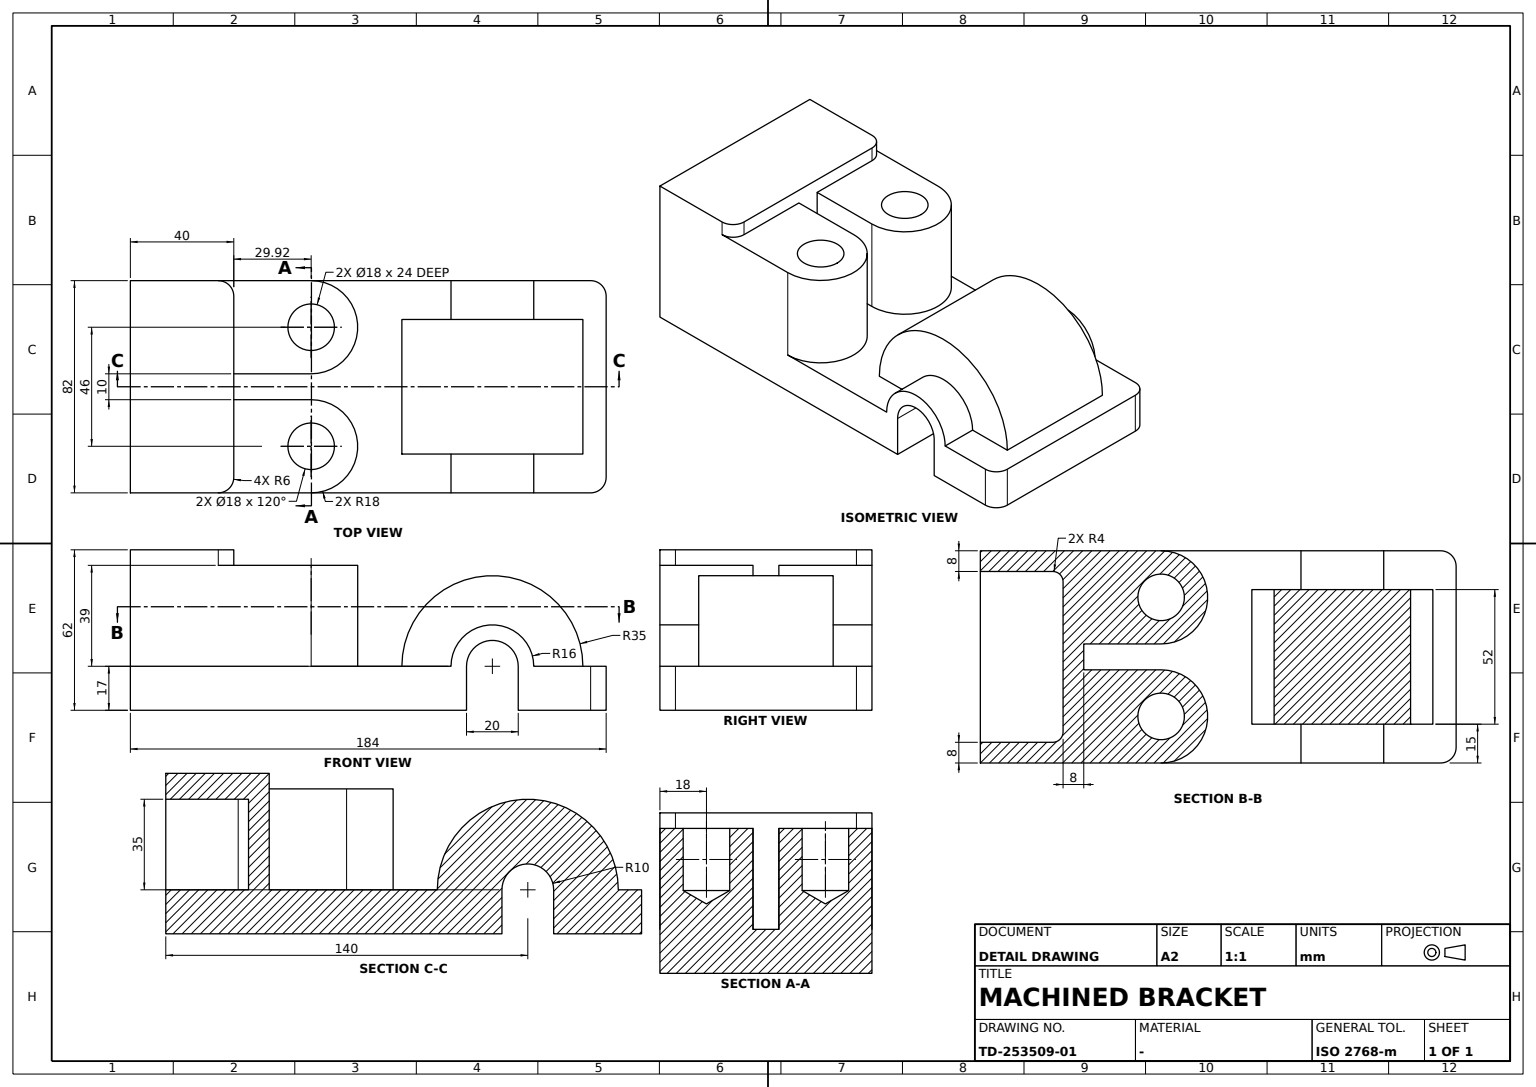
ISO-10303-21;
HEADER;
FILE_DESCRIPTION((''),'2;1');
FILE_NAME('','',(''),(''),'','','');
FILE_SCHEMA(('AUTOMOTIVE_DESIGN'));
ENDSEC;
DATA;
#1=APPLICATION_CONTEXT('');
#2=PRODUCT_CONTEXT('',#1,'mechanical');
#3=PRODUCT('','','',(#2));
#4=PRODUCT_DEFINITION_FORMATION('','',#3);
#5=PRODUCT_DEFINITION_CONTEXT('',#1,'design');
#6=PRODUCT_DEFINITION('','',#4,#5);
#7=PRODUCT_DEFINITION_SHAPE('','',#6);
#8=(LENGTH_UNIT()NAMED_UNIT(*)SI_UNIT(.MILLI.,.METRE.));
#9=(NAMED_UNIT(*)PLANE_ANGLE_UNIT()SI_UNIT($,.RADIAN.));
#10=(NAMED_UNIT(*)SI_UNIT($,.STERADIAN.)SOLID_ANGLE_UNIT());
#11=UNCERTAINTY_MEASURE_WITH_UNIT(LENGTH_MEASURE(0.005),#8,'distance_accuracy_value','');
#12=(GEOMETRIC_REPRESENTATION_CONTEXT(3)GLOBAL_UNCERTAINTY_ASSIGNED_CONTEXT((#11))GLOBAL_UNIT_ASSIGNED_CONTEXT((#8,#9,#10))REPRESENTATION_CONTEXT('',''));
#13=CARTESIAN_POINT('',(10.,-41.,0.));
#14=VERTEX_POINT('',#13);
#15=CARTESIAN_POINT('',(10.,-41.,-17.));
#16=VERTEX_POINT('',#15);
#17=DIRECTION('',(0.,0.,-1.));
#18=VECTOR('',#17,1000.);
#19=LINE('',#13,#18);
#20=EDGE_CURVE('',#14,#16,#19,.T.);
#21=ORIENTED_EDGE('',*,*,#20,.F.);
#22=CARTESIAN_POINT('',(10.,41.,0.));
#23=VERTEX_POINT('',#22);
#24=CARTESIAN_POINT('',(10.,0.,0.));
#25=DIRECTION('',(0.,1.,0.));
#26=VECTOR('',#25,1000.);
#27=LINE('',#24,#26);
#28=EDGE_CURVE('',#14,#23,#27,.T.);
#29=ORIENTED_EDGE('',*,*,#28,.T.);
#30=CARTESIAN_POINT('',(10.,41.,-17.));
#31=VERTEX_POINT('',#30);
#32=LINE('',#22,#18);
#33=EDGE_CURVE('',#23,#31,#32,.T.);
#34=ORIENTED_EDGE('',*,*,#33,.T.);
#35=CARTESIAN_POINT('',(10.,0.,-17.));
#36=LINE('',#35,#26);
#37=EDGE_CURVE('',#16,#31,#36,.T.);
#38=ORIENTED_EDGE('',*,*,#37,.F.);
#39=EDGE_LOOP('',(#21,#29,#34,#38));
#40=FACE_BOUND('',#39,.T.);
#41=DIRECTION('',(1.,0.,0.));
#42=AXIS2_PLACEMENT_3D('',#24,#41,#17);
#43=PLANE('',#42);
#44=ADVANCED_FACE('',(#40),#43,.F.);
#45=CARTESIAN_POINT('',(-16.,26.,0.));
#46=VERTEX_POINT('',#45);
#47=CARTESIAN_POINT('',(-16.,41.,0.));
#48=VERTEX_POINT('',#47);
#49=LINE('',#45,#26);
#50=EDGE_CURVE('',#46,#48,#49,.T.);
#51=ORIENTED_EDGE('',*,*,#50,.F.);
#52=CARTESIAN_POINT('',(16.,26.,0.));
#53=VERTEX_POINT('',#52);
#54=CARTESIAN_POINT('',(0.,26.,0.));
#55=DIRECTION('',(0.,0.,1.));
#56=AXIS2_PLACEMENT_3D('',#54,#25,#55);
#57=CIRCLE('',#56,16.);
#58=EDGE_CURVE('',#46,#53,#57,.T.);
#59=ORIENTED_EDGE('',*,*,#58,.T.);
#60=CARTESIAN_POINT('',(16.,41.,0.));
#61=VERTEX_POINT('',#60);
#62=LINE('',#52,#26);
#63=EDGE_CURVE('',#53,#61,#62,.T.);
#64=ORIENTED_EDGE('',*,*,#63,.T.);
#65=CARTESIAN_POINT('',(0.,41.,0.));
#66=AXIS2_PLACEMENT_3D('',#65,#25,#55);
#67=CIRCLE('',#66,16.);
#68=EDGE_CURVE('',#48,#61,#67,.T.);
#69=ORIENTED_EDGE('',*,*,#68,.F.);
#70=EDGE_LOOP('',(#51,#59,#64,#69));
#71=FACE_BOUND('',#70,.T.);
#72=CARTESIAN_POINT('',(0.,0.,0.));
#73=DIRECTION('',(-1.,0.,0.));
#74=AXIS2_PLACEMENT_3D('',#72,#25,#73);
#75=CYLINDRICAL_SURFACE('',#74,16.);
#76=ADVANCED_FACE('',(#71),#75,.T.);
#77=CARTESIAN_POINT('',(-70.080651,-5.,39.));
#78=VERTEX_POINT('',#77);
#79=CARTESIAN_POINT('',(-100.,-5.,39.));
#80=VERTEX_POINT('',#79);
#81=CARTESIAN_POINT('',(0.,-5.,39.));
#82=VECTOR('',#73,1000.);
#83=LINE('',#81,#82);
#84=EDGE_CURVE('',#78,#80,#83,.T.);
#85=ORIENTED_EDGE('',*,*,#84,.F.);
#86=CARTESIAN_POINT('',(-70.080651,-5.,0.));
#87=VERTEX_POINT('',#86);
#88=CARTESIAN_POINT('',(-70.080651,-5.,19.5));
#89=VECTOR('',#55,1000.);
#90=LINE('',#88,#89);
#91=EDGE_CURVE('',#87,#78,#90,.T.);
#92=ORIENTED_EDGE('',*,*,#91,.F.);
#93=CARTESIAN_POINT('',(-100.,-5.,0.));
#94=VERTEX_POINT('',#93);
#95=LINE('',#86,#82);
#96=EDGE_CURVE('',#87,#94,#95,.T.);
#97=ORIENTED_EDGE('',*,*,#96,.T.);
#98=CARTESIAN_POINT('',(-100.,-5.,45.));
#99=LINE('',#98,#89);
#100=EDGE_CURVE('',#94,#80,#99,.T.);
#101=ORIENTED_EDGE('',*,*,#100,.T.);
#102=EDGE_LOOP('',(#85,#92,#97,#101));
#103=FACE_BOUND('',#102,.T.);
#104=AXIS2_PLACEMENT_3D('',#86,#25,#73);
#105=PLANE('',#104);
#106=ADVANCED_FACE('',(#103),#105,.T.);
#107=CARTESIAN_POINT('',(38.,41.,-17.));
#108=VERTEX_POINT('',#107);
#109=CARTESIAN_POINT('',(0.,41.,-17.));
#110=VECTOR('',#41,1000.);
#111=LINE('',#109,#110);
#112=EDGE_CURVE('',#31,#108,#111,.T.);
#113=ORIENTED_EDGE('',*,*,#112,.F.);
#114=ORIENTED_EDGE('',*,*,#33,.F.);
#115=CARTESIAN_POINT('',(-10.,41.,0.));
#116=VERTEX_POINT('',#115);
#117=CIRCLE('',#66,10.);
#118=EDGE_CURVE('',#116,#23,#117,.T.);
#119=ORIENTED_EDGE('',*,*,#118,.F.);
#120=CARTESIAN_POINT('',(-10.,41.,-17.));
#121=VERTEX_POINT('',#120);
#122=LINE('',#115,#18);
#123=EDGE_CURVE('',#116,#121,#122,.T.);
#124=ORIENTED_EDGE('',*,*,#123,.T.);
#125=CARTESIAN_POINT('',(-140.,41.,-17.));
#126=VERTEX_POINT('',#125);
#127=EDGE_CURVE('',#126,#121,#111,.T.);
#128=ORIENTED_EDGE('',*,*,#127,.F.);
#129=CARTESIAN_POINT('',(-140.,41.,45.));
#130=VERTEX_POINT('',#129);
#131=CARTESIAN_POINT('',(-140.,41.,0.));
#132=LINE('',#131,#89);
#133=EDGE_CURVE('',#126,#130,#132,.T.);
#134=ORIENTED_EDGE('',*,*,#133,.T.);
#135=CARTESIAN_POINT('',(-106.,41.,45.));
#136=VERTEX_POINT('',#135);
#137=CARTESIAN_POINT('',(0.,41.,45.));
#138=LINE('',#137,#110);
#139=EDGE_CURVE('',#130,#136,#138,.T.);
#140=ORIENTED_EDGE('',*,*,#139,.T.);
#141=CARTESIAN_POINT('',(-106.,41.,39.));
#142=VERTEX_POINT('',#141);
#143=CARTESIAN_POINT('',(-106.,41.,40.));
#144=LINE('',#143,#89);
#145=EDGE_CURVE('',#136,#142,#144,.F.);
#146=ORIENTED_EDGE('',*,*,#145,.T.);
#147=CARTESIAN_POINT('',(-70.080651,41.,39.));
#148=VERTEX_POINT('',#147);
#149=CARTESIAN_POINT('',(0.,41.,39.));
#150=LINE('',#149,#82);
#151=EDGE_CURVE('',#148,#142,#150,.T.);
#152=ORIENTED_EDGE('',*,*,#151,.F.);
#153=CARTESIAN_POINT('',(-70.080651,41.,0.));
#154=VERTEX_POINT('',#153);
#155=CARTESIAN_POINT('',(-70.080651,41.,19.5));
#156=LINE('',#155,#89);
#157=EDGE_CURVE('',#154,#148,#156,.T.);
#158=ORIENTED_EDGE('',*,*,#157,.F.);
#159=LINE('',#65,#82);
#160=EDGE_CURVE('',#48,#154,#159,.T.);
#161=ORIENTED_EDGE('',*,*,#160,.F.);
#162=ORIENTED_EDGE('',*,*,#68,.T.);
#163=CARTESIAN_POINT('',(38.,41.,0.));
#164=VERTEX_POINT('',#163);
#165=EDGE_CURVE('',#164,#61,#159,.T.);
#166=ORIENTED_EDGE('',*,*,#165,.F.);
#167=CARTESIAN_POINT('',(38.,41.,14.));
#168=LINE('',#167,#18);
#169=EDGE_CURVE('',#164,#108,#168,.T.);
#170=ORIENTED_EDGE('',*,*,#169,.T.);
#171=EDGE_LOOP('',(#113,#114,#119,#124,#128,#134,#140,#146,#152,#158,#161,#162,#166,#170));
#172=FACE_BOUND('',#171,.T.);
#173=AXIS2_PLACEMENT_3D('',#65,#25,#73);
#174=PLANE('',#173);
#175=ADVANCED_FACE('',(#172),#174,.T.);
#176=CARTESIAN_POINT('',(-140.,-33.,35.));
#177=VERTEX_POINT('',#176);
#178=CARTESIAN_POINT('',(-140.,33.,35.));
#179=VERTEX_POINT('',#178);
#180=CARTESIAN_POINT('',(-140.,0.,35.));
#181=LINE('',#180,#26);
#182=EDGE_CURVE('',#177,#179,#181,.T.);
#183=ORIENTED_EDGE('',*,*,#182,.T.);
#184=CARTESIAN_POINT('',(-112.,33.,35.));
#185=VERTEX_POINT('',#184);
#186=LINE('',#178,#110);
#187=EDGE_CURVE('',#179,#185,#186,.T.);
#188=ORIENTED_EDGE('',*,*,#187,.T.);
#189=CARTESIAN_POINT('',(-108.,29.,35.));
#190=VERTEX_POINT('',#189);
#191=CARTESIAN_POINT('',(-112.,29.,35.));
#192=AXIS2_PLACEMENT_3D('',#191,#55,#41);
#193=CIRCLE('',#192,4.);
#194=EDGE_CURVE('',#190,#185,#193,.T.);
#195=ORIENTED_EDGE('',*,*,#194,.F.);
#196=CARTESIAN_POINT('',(-108.,-29.,35.));
#197=VERTEX_POINT('',#196);
#198=DIRECTION('',(0.,-1.,0.));
#199=VECTOR('',#198,1000.);
#200=LINE('',#189,#199);
#201=EDGE_CURVE('',#190,#197,#200,.T.);
#202=ORIENTED_EDGE('',*,*,#201,.T.);
#203=CARTESIAN_POINT('',(-112.,-33.,35.));
#204=VERTEX_POINT('',#203);
#205=CARTESIAN_POINT('',(-112.,-29.,35.));
#206=AXIS2_PLACEMENT_3D('',#205,#55,#41);
#207=CIRCLE('',#206,4.);
#208=EDGE_CURVE('',#204,#197,#207,.T.);
#209=ORIENTED_EDGE('',*,*,#208,.F.);
#210=CARTESIAN_POINT('',(0.,-33.,35.));
#211=LINE('',#210,#110);
#212=EDGE_CURVE('',#177,#204,#211,.T.);
#213=ORIENTED_EDGE('',*,*,#212,.F.);
#214=EDGE_LOOP('',(#183,#188,#195,#202,#209,#213));
#215=FACE_BOUND('',#214,.T.);
#216=CARTESIAN_POINT('',(0.,0.,35.));
#217=AXIS2_PLACEMENT_3D('',#216,#55,#41);
#218=PLANE('',#217);
#219=ADVANCED_FACE('',(#215),#218,.F.);
#220=CARTESIAN_POINT('',(-140.,-41.,45.));
#221=VERTEX_POINT('',#220);
#222=CARTESIAN_POINT('',(-106.,-41.,45.));
#223=VERTEX_POINT('',#222);
#224=CARTESIAN_POINT('',(0.,-41.,45.));
#225=LINE('',#224,#110);
#226=EDGE_CURVE('',#221,#223,#225,.T.);
#227=ORIENTED_EDGE('',*,*,#226,.F.);
#228=CARTESIAN_POINT('',(-140.,-41.,-17.));
#229=VERTEX_POINT('',#228);
#230=CARTESIAN_POINT('',(-140.,-41.,0.));
#231=LINE('',#230,#89);
#232=EDGE_CURVE('',#229,#221,#231,.T.);
#233=ORIENTED_EDGE('',*,*,#232,.F.);
#234=CARTESIAN_POINT('',(-10.,-41.,-17.));
#235=VERTEX_POINT('',#234);
#236=CARTESIAN_POINT('',(0.,-41.,-17.));
#237=LINE('',#236,#110);
#238=EDGE_CURVE('',#229,#235,#237,.T.);
#239=ORIENTED_EDGE('',*,*,#238,.T.);
#240=CARTESIAN_POINT('',(-10.,-41.,0.));
#241=VERTEX_POINT('',#240);
#242=LINE('',#240,#18);
#243=EDGE_CURVE('',#241,#235,#242,.T.);
#244=ORIENTED_EDGE('',*,*,#243,.F.);
#245=CARTESIAN_POINT('',(0.,-41.,0.));
#246=AXIS2_PLACEMENT_3D('',#245,#25,#55);
#247=CIRCLE('',#246,10.);
#248=EDGE_CURVE('',#241,#14,#247,.T.);
#249=ORIENTED_EDGE('',*,*,#248,.T.);
#250=ORIENTED_EDGE('',*,*,#20,.T.);
#251=CARTESIAN_POINT('',(38.,-41.,-17.));
#252=VERTEX_POINT('',#251);
#253=EDGE_CURVE('',#16,#252,#237,.T.);
#254=ORIENTED_EDGE('',*,*,#253,.T.);
#255=CARTESIAN_POINT('',(38.,-41.,0.));
#256=VERTEX_POINT('',#255);
#257=CARTESIAN_POINT('',(38.,-41.,14.));
#258=LINE('',#257,#18);
#259=EDGE_CURVE('',#256,#252,#258,.T.);
#260=ORIENTED_EDGE('',*,*,#259,.F.);
#261=CARTESIAN_POINT('',(16.,-41.,0.));
#262=VERTEX_POINT('',#261);
#263=LINE('',#245,#82);
#264=EDGE_CURVE('',#256,#262,#263,.T.);
#265=ORIENTED_EDGE('',*,*,#264,.T.);
#266=CARTESIAN_POINT('',(-16.,-41.,0.));
#267=VERTEX_POINT('',#266);
#268=CIRCLE('',#246,16.);
#269=EDGE_CURVE('',#267,#262,#268,.T.);
#270=ORIENTED_EDGE('',*,*,#269,.F.);
#271=CARTESIAN_POINT('',(-70.080651,-41.,0.));
#272=VERTEX_POINT('',#271);
#273=EDGE_CURVE('',#267,#272,#263,.T.);
#274=ORIENTED_EDGE('',*,*,#273,.T.);
#275=CARTESIAN_POINT('',(-70.080651,-41.,39.));
#276=VERTEX_POINT('',#275);
#277=CARTESIAN_POINT('',(-70.080651,-41.,19.5));
#278=LINE('',#277,#89);
#279=EDGE_CURVE('',#272,#276,#278,.T.);
#280=ORIENTED_EDGE('',*,*,#279,.T.);
#281=CARTESIAN_POINT('',(-106.,-41.,39.));
#282=VERTEX_POINT('',#281);
#283=CARTESIAN_POINT('',(0.,-41.,39.));
#284=LINE('',#283,#110);
#285=EDGE_CURVE('',#282,#276,#284,.T.);
#286=ORIENTED_EDGE('',*,*,#285,.F.);
#287=CARTESIAN_POINT('',(-106.,-41.,40.));
#288=LINE('',#287,#89);
#289=EDGE_CURVE('',#223,#282,#288,.F.);
#290=ORIENTED_EDGE('',*,*,#289,.F.);
#291=EDGE_LOOP('',(#227,#233,#239,#244,#249,#250,#254,#260,#265,#270,#274,#280,#286,#290));
#292=FACE_BOUND('',#291,.T.);
#293=AXIS2_PLACEMENT_3D('',#245,#25,#73);
#294=PLANE('',#293);
#295=ADVANCED_FACE('',(#292),#294,.F.);
#296=CARTESIAN_POINT('',(-100.,-35.,45.));
#297=VERTEX_POINT('',#296);
#298=CARTESIAN_POINT('',(-106.,-35.,45.));
#299=AXIS2_PLACEMENT_3D('',#298,#55,#41);
#300=CIRCLE('',#299,6.);
#301=EDGE_CURVE('',#223,#297,#300,.T.);
#302=ORIENTED_EDGE('',*,*,#301,.F.);
#303=ORIENTED_EDGE('',*,*,#289,.T.);
#304=CARTESIAN_POINT('',(-100.,-35.,39.));
#305=VERTEX_POINT('',#304);
#306=CARTESIAN_POINT('',(-106.,-35.,39.));
#307=AXIS2_PLACEMENT_3D('',#306,#55,#41);
#308=CIRCLE('',#307,6.);
#309=EDGE_CURVE('',#282,#305,#308,.T.);
#310=ORIENTED_EDGE('',*,*,#309,.T.);
#311=CARTESIAN_POINT('',(-100.,-35.,40.));
#312=LINE('',#311,#89);
#313=EDGE_CURVE('',#297,#305,#312,.F.);
#314=ORIENTED_EDGE('',*,*,#313,.F.);
#315=EDGE_LOOP('',(#302,#303,#310,#314));
#316=FACE_BOUND('',#315,.T.);
#317=CARTESIAN_POINT('',(-106.,-35.,40.));
#318=AXIS2_PLACEMENT_3D('',#317,#55,#41);
#319=CYLINDRICAL_SURFACE('',#318,6.);
#320=ADVANCED_FACE('',(#316),#319,.T.);
#321=CARTESIAN_POINT('',(44.,-35.,0.));
#322=VERTEX_POINT('',#321);
#323=CARTESIAN_POINT('',(44.,35.,0.));
#324=VERTEX_POINT('',#323);
#325=CARTESIAN_POINT('',(44.,0.,0.));
#326=LINE('',#325,#26);
#327=EDGE_CURVE('',#322,#324,#326,.T.);
#328=ORIENTED_EDGE('',*,*,#327,.T.);
#329=CARTESIAN_POINT('',(38.,35.,0.));
#330=AXIS2_PLACEMENT_3D('',#329,#17,#73);
#331=CIRCLE('',#330,6.);
#332=EDGE_CURVE('',#164,#324,#331,.T.);
#333=ORIENTED_EDGE('',*,*,#332,.F.);
#334=ORIENTED_EDGE('',*,*,#165,.T.);
#335=ORIENTED_EDGE('',*,*,#63,.F.);
#336=CARTESIAN_POINT('',(35.,26.,0.));
#337=VERTEX_POINT('',#336);
#338=CARTESIAN_POINT('',(44.,26.,0.));
#339=LINE('',#338,#110);
#340=EDGE_CURVE('',#53,#337,#339,.T.);
#341=ORIENTED_EDGE('',*,*,#340,.T.);
#342=CARTESIAN_POINT('',(35.,-26.,0.));
#343=VERTEX_POINT('',#342);
#344=LINE('',#342,#26);
#345=EDGE_CURVE('',#343,#337,#344,.T.);
#346=ORIENTED_EDGE('',*,*,#345,.F.);
#347=CARTESIAN_POINT('',(16.,-26.,0.));
#348=VERTEX_POINT('',#347);
#349=CARTESIAN_POINT('',(44.,-26.,0.));
#350=LINE('',#349,#110);
#351=EDGE_CURVE('',#348,#343,#350,.T.);
#352=ORIENTED_EDGE('',*,*,#351,.F.);
#353=LINE('',#261,#26);
#354=EDGE_CURVE('',#262,#348,#353,.T.);
#355=ORIENTED_EDGE('',*,*,#354,.F.);
#356=ORIENTED_EDGE('',*,*,#264,.F.);
#357=CARTESIAN_POINT('',(38.,-35.,0.));
#358=AXIS2_PLACEMENT_3D('',#357,#17,#73);
#359=CIRCLE('',#358,6.);
#360=EDGE_CURVE('',#322,#256,#359,.T.);
#361=ORIENTED_EDGE('',*,*,#360,.F.);
#362=EDGE_LOOP('',(#328,#333,#334,#335,#341,#346,#352,#355,#356,#361));
#363=FACE_BOUND('',#362,.T.);
#364=AXIS2_PLACEMENT_3D('',#325,#17,#73);
#365=PLANE('',#364);
#366=ADVANCED_FACE('',(#363),#365,.F.);
#367=ORIENTED_EDGE('',*,*,#58,.F.);
#368=CARTESIAN_POINT('',(-35.,26.,0.));
#369=VERTEX_POINT('',#368);
#370=LINE('',#54,#82);
#371=EDGE_CURVE('',#46,#369,#370,.T.);
#372=ORIENTED_EDGE('',*,*,#371,.T.);
#373=CIRCLE('',#56,35.);
#374=EDGE_CURVE('',#369,#337,#373,.T.);
#375=ORIENTED_EDGE('',*,*,#374,.T.);
#376=ORIENTED_EDGE('',*,*,#340,.F.);
#377=EDGE_LOOP('',(#367,#372,#375,#376));
#378=FACE_BOUND('',#377,.T.);
#379=AXIS2_PLACEMENT_3D('',#54,#25,#73);
#380=PLANE('',#379);
#381=ADVANCED_FACE('',(#378),#380,.T.);
#382=ORIENTED_EDGE('',*,*,#212,.T.);
#383=CARTESIAN_POINT('',(-112.,-33.,0.));
#384=VERTEX_POINT('',#383);
#385=CARTESIAN_POINT('',(-112.,-33.,22.5));
#386=LINE('',#385,#89);
#387=EDGE_CURVE('',#204,#384,#386,.F.);
#388=ORIENTED_EDGE('',*,*,#387,.T.);
#389=CARTESIAN_POINT('',(-140.,-33.,0.));
#390=VERTEX_POINT('',#389);
#391=CARTESIAN_POINT('',(44.,-33.,0.));
#392=LINE('',#391,#82);
#393=EDGE_CURVE('',#384,#390,#392,.T.);
#394=ORIENTED_EDGE('',*,*,#393,.T.);
#395=CARTESIAN_POINT('',(-140.,-33.,45.));
#396=LINE('',#395,#18);
#397=EDGE_CURVE('',#177,#390,#396,.T.);
#398=ORIENTED_EDGE('',*,*,#397,.F.);
#399=EDGE_LOOP('',(#382,#388,#394,#398));
#400=FACE_BOUND('',#399,.T.);
#401=CARTESIAN_POINT('',(-112.,-33.,45.));
#402=AXIS2_PLACEMENT_3D('',#401,#198,#73);
#403=PLANE('',#402);
#404=ADVANCED_FACE('',(#400),#403,.F.);
#405=CARTESIAN_POINT('',(-108.,29.,0.));
#406=VERTEX_POINT('',#405);
#407=CARTESIAN_POINT('',(-108.,29.,22.5));
#408=LINE('',#407,#89);
#409=EDGE_CURVE('',#190,#406,#408,.F.);
#410=ORIENTED_EDGE('',*,*,#409,.F.);
#411=ORIENTED_EDGE('',*,*,#194,.T.);
#412=CARTESIAN_POINT('',(-112.,33.,0.));
#413=VERTEX_POINT('',#412);
#414=CARTESIAN_POINT('',(-112.,33.,22.5));
#415=LINE('',#414,#89);
#416=EDGE_CURVE('',#185,#413,#415,.F.);
#417=ORIENTED_EDGE('',*,*,#416,.T.);
#418=CARTESIAN_POINT('',(-112.,29.,0.));
#419=AXIS2_PLACEMENT_3D('',#418,#17,#73);
#420=CIRCLE('',#419,4.);
#421=EDGE_CURVE('',#406,#413,#420,.F.);
#422=ORIENTED_EDGE('',*,*,#421,.F.);
#423=EDGE_LOOP('',(#410,#411,#417,#422));
#424=FACE_BOUND('',#423,.T.);
#425=CARTESIAN_POINT('',(-112.,29.,22.5));
#426=AXIS2_PLACEMENT_3D('',#425,#55,#41);
#427=CYLINDRICAL_SURFACE('',#426,4.);
#428=ADVANCED_FACE('',(#424),#427,.F.);
#429=ORIENTED_EDGE('',*,*,#397,.T.);
#430=CARTESIAN_POINT('',(-140.,33.,0.));
#431=VERTEX_POINT('',#430);
#432=CARTESIAN_POINT('',(-140.,0.,0.));
#433=LINE('',#432,#199);
#434=EDGE_CURVE('',#431,#390,#433,.T.);
#435=ORIENTED_EDGE('',*,*,#434,.F.);
#436=CARTESIAN_POINT('',(-140.,33.,-17.));
#437=LINE('',#436,#18);
#438=EDGE_CURVE('',#179,#431,#437,.T.);
#439=ORIENTED_EDGE('',*,*,#438,.F.);
#440=ORIENTED_EDGE('',*,*,#182,.F.);
#441=EDGE_LOOP('',(#429,#435,#439,#440));
#442=FACE_BOUND('',#441,.T.);
#443=CARTESIAN_POINT('',(-140.,0.,-17.));
#444=LINE('',#443,#26);
#445=EDGE_CURVE('',#229,#126,#444,.T.);
#446=ORIENTED_EDGE('',*,*,#445,.F.);
#447=ORIENTED_EDGE('',*,*,#232,.T.);
#448=CARTESIAN_POINT('',(-140.,0.,45.));
#449=LINE('',#448,#26);
#450=EDGE_CURVE('',#221,#130,#449,.T.);
#451=ORIENTED_EDGE('',*,*,#450,.T.);
#452=ORIENTED_EDGE('',*,*,#133,.F.);
#453=EDGE_LOOP('',(#446,#447,#451,#452));
#454=FACE_BOUND('',#453,.T.);
#455=AXIS2_PLACEMENT_3D('',#443,#73,#55);
#456=PLANE('',#455);
#457=ADVANCED_FACE('',(#442,#454),#456,.T.);
#458=CARTESIAN_POINT('',(-100.,35.,45.));
#459=VERTEX_POINT('',#458);
#460=CARTESIAN_POINT('',(-100.,35.,39.));
#461=VERTEX_POINT('',#460);
#462=CARTESIAN_POINT('',(-100.,35.,40.));
#463=LINE('',#462,#89);
#464=EDGE_CURVE('',#459,#461,#463,.F.);
#465=ORIENTED_EDGE('',*,*,#464,.T.);
#466=CARTESIAN_POINT('',(-106.,35.,39.));
#467=AXIS2_PLACEMENT_3D('',#466,#55,#41);
#468=CIRCLE('',#467,6.);
#469=EDGE_CURVE('',#461,#142,#468,.T.);
#470=ORIENTED_EDGE('',*,*,#469,.T.);
#471=ORIENTED_EDGE('',*,*,#145,.F.);
#472=CARTESIAN_POINT('',(-106.,35.,45.));
#473=AXIS2_PLACEMENT_3D('',#472,#55,#41);
#474=CIRCLE('',#473,6.);
#475=EDGE_CURVE('',#459,#136,#474,.T.);
#476=ORIENTED_EDGE('',*,*,#475,.F.);
#477=EDGE_LOOP('',(#465,#470,#471,#476));
#478=FACE_BOUND('',#477,.T.);
#479=CARTESIAN_POINT('',(-106.,35.,40.));
#480=AXIS2_PLACEMENT_3D('',#479,#55,#41);
#481=CYLINDRICAL_SURFACE('',#480,6.);
#482=ADVANCED_FACE('',(#478),#481,.T.);
#483=CARTESIAN_POINT('',(-61.080651,-23.,15.));
#484=VERTEX_POINT('',#483);
#485=CARTESIAN_POINT('',(-70.080651,-23.,15.));
#486=AXIS2_PLACEMENT_3D('',#485,#55,#41);
#487=CIRCLE('',#486,9.);
#488=EDGE_CURVE('',#484,#484,#487,.F.);
#489=ORIENTED_EDGE('',*,*,#488,.F.);
#490=EDGE_LOOP('',(#489));
#491=FACE_BOUND('',#490,.T.);
#492=CARTESIAN_POINT('',(-70.080651,-23.,9.803848));
#493=VERTEX_POINT('',#492);
#494=VERTEX_LOOP('',#493);
#495=FACE_BOUND('',#494,.T.);
#496=AXIS2_PLACEMENT_3D('',#492,#55,#41);
#497=CONICAL_SURFACE('',#496,0.,1.047197551);
#498=ADVANCED_FACE('',(#491,#495),#497,.F.);
#499=ORIENTED_EDGE('',*,*,#243,.T.);
#500=CARTESIAN_POINT('',(-10.,0.,-17.));
#501=LINE('',#500,#26);
#502=EDGE_CURVE('',#235,#121,#501,.T.);
#503=ORIENTED_EDGE('',*,*,#502,.T.);
#504=ORIENTED_EDGE('',*,*,#123,.F.);
#505=CARTESIAN_POINT('',(-10.,0.,0.));
#506=LINE('',#505,#26);
#507=EDGE_CURVE('',#241,#116,#506,.T.);
#508=ORIENTED_EDGE('',*,*,#507,.F.);
#509=EDGE_LOOP('',(#499,#503,#504,#508));
#510=FACE_BOUND('',#509,.T.);
#511=AXIS2_PLACEMENT_3D('',#505,#41,#17);
#512=PLANE('',#511);
#513=ADVANCED_FACE('',(#510),#512,.T.);
#514=ORIENTED_EDGE('',*,*,#332,.T.);
#515=CARTESIAN_POINT('',(44.,35.,-17.));
#516=VERTEX_POINT('',#515);
#517=CARTESIAN_POINT('',(44.,35.,14.));
#518=LINE('',#517,#18);
#519=EDGE_CURVE('',#324,#516,#518,.T.);
#520=ORIENTED_EDGE('',*,*,#519,.T.);
#521=CARTESIAN_POINT('',(38.,35.,-17.));
#522=AXIS2_PLACEMENT_3D('',#521,#55,#41);
#523=CIRCLE('',#522,6.);
#524=EDGE_CURVE('',#516,#108,#523,.T.);
#525=ORIENTED_EDGE('',*,*,#524,.T.);
#526=ORIENTED_EDGE('',*,*,#169,.F.);
#527=EDGE_LOOP('',(#514,#520,#525,#526));
#528=FACE_BOUND('',#527,.T.);
#529=CARTESIAN_POINT('',(38.,35.,14.));
#530=AXIS2_PLACEMENT_3D('',#529,#17,#41);
#531=CYLINDRICAL_SURFACE('',#530,6.);
#532=ADVANCED_FACE('',(#528),#531,.T.);
#533=CARTESIAN_POINT('',(-70.080651,5.,0.));
#534=VERTEX_POINT('',#533);
#535=CARTESIAN_POINT('',(-70.080651,23.,0.));
#536=AXIS2_PLACEMENT_3D('',#535,#17,#73);
#537=CIRCLE('',#536,18.);
#538=EDGE_CURVE('',#534,#154,#537,.F.);
#539=ORIENTED_EDGE('',*,*,#538,.T.);
#540=ORIENTED_EDGE('',*,*,#157,.T.);
#541=CARTESIAN_POINT('',(-70.080651,5.,39.));
#542=VERTEX_POINT('',#541);
#543=CARTESIAN_POINT('',(-70.080651,23.,39.));
#544=AXIS2_PLACEMENT_3D('',#543,#55,#41);
#545=CIRCLE('',#544,18.);
#546=EDGE_CURVE('',#542,#148,#545,.T.);
#547=ORIENTED_EDGE('',*,*,#546,.F.);
#548=CARTESIAN_POINT('',(-70.080651,5.,19.5));
#549=LINE('',#548,#89);
#550=EDGE_CURVE('',#534,#542,#549,.T.);
#551=ORIENTED_EDGE('',*,*,#550,.F.);
#552=EDGE_LOOP('',(#539,#540,#547,#551));
#553=FACE_BOUND('',#552,.T.);
#554=CARTESIAN_POINT('',(-70.080651,23.,19.5));
#555=AXIS2_PLACEMENT_3D('',#554,#55,#41);
#556=CYLINDRICAL_SURFACE('',#555,18.);
#557=ADVANCED_FACE('',(#553),#556,.T.);
#558=CARTESIAN_POINT('',(-61.080651,23.,15.));
#559=VERTEX_POINT('',#558);
#560=CARTESIAN_POINT('',(-70.080651,23.,15.));
#561=AXIS2_PLACEMENT_3D('',#560,#55,#41);
#562=CIRCLE('',#561,9.);
#563=EDGE_CURVE('',#559,#559,#562,.F.);
#564=ORIENTED_EDGE('',*,*,#563,.T.);
#565=EDGE_LOOP('',(#564));
#566=FACE_BOUND('',#565,.T.);
#567=CARTESIAN_POINT('',(-61.080651,23.,39.));
#568=VERTEX_POINT('',#567);
#569=CIRCLE('',#544,9.);
#570=EDGE_CURVE('',#568,#568,#569,.T.);
#571=ORIENTED_EDGE('',*,*,#570,.T.);
#572=EDGE_LOOP('',(#571));
#573=FACE_BOUND('',#572,.T.);
#574=CARTESIAN_POINT('',(-70.080651,23.,38.9));
#575=AXIS2_PLACEMENT_3D('',#574,#17,#41);
#576=CYLINDRICAL_SURFACE('',#575,9.);
#577=ADVANCED_FACE('',(#566,#573),#576,.F.);
#578=ORIENTED_EDGE('',*,*,#570,.F.);
#579=EDGE_LOOP('',(#578));
#580=FACE_BOUND('',#579,.T.);
#581=ORIENTED_EDGE('',*,*,#469,.F.);
#582=CARTESIAN_POINT('',(-100.,5.,39.));
#583=VERTEX_POINT('',#582);
#584=CARTESIAN_POINT('',(-100.,0.,39.));
#585=LINE('',#584,#26);
#586=EDGE_CURVE('',#583,#461,#585,.T.);
#587=ORIENTED_EDGE('',*,*,#586,.F.);
#588=CARTESIAN_POINT('',(0.,5.,39.));
#589=LINE('',#588,#82);
#590=EDGE_CURVE('',#542,#583,#589,.T.);
#591=ORIENTED_EDGE('',*,*,#590,.F.);
#592=ORIENTED_EDGE('',*,*,#546,.T.);
#593=ORIENTED_EDGE('',*,*,#151,.T.);
#594=EDGE_LOOP('',(#581,#587,#591,#592,#593));
#595=FACE_BOUND('',#594,.T.);
#596=CARTESIAN_POINT('',(0.,0.,39.));
#597=AXIS2_PLACEMENT_3D('',#596,#55,#41);
#598=PLANE('',#597);
#599=ADVANCED_FACE('',(#580,#595),#598,.T.);
#600=ORIENTED_EDGE('',*,*,#507,.T.);
#601=ORIENTED_EDGE('',*,*,#118,.T.);
#602=ORIENTED_EDGE('',*,*,#28,.F.);
#603=ORIENTED_EDGE('',*,*,#248,.F.);
#604=EDGE_LOOP('',(#600,#601,#602,#603));
#605=FACE_BOUND('',#604,.T.);
#606=CYLINDRICAL_SURFACE('',#74,10.);
#607=ADVANCED_FACE('',(#605),#606,.F.);
#608=CARTESIAN_POINT('',(-61.080651,-23.,39.));
#609=VERTEX_POINT('',#608);
#610=CARTESIAN_POINT('',(-70.080651,-23.,39.));
#611=AXIS2_PLACEMENT_3D('',#610,#55,#41);
#612=CIRCLE('',#611,9.);
#613=EDGE_CURVE('',#609,#609,#612,.T.);
#614=ORIENTED_EDGE('',*,*,#613,.T.);
#615=EDGE_LOOP('',(#614));
#616=FACE_BOUND('',#615,.T.);
#617=ORIENTED_EDGE('',*,*,#488,.T.);
#618=EDGE_LOOP('',(#617));
#619=FACE_BOUND('',#618,.T.);
#620=CARTESIAN_POINT('',(-70.080651,-23.,38.9));
#621=AXIS2_PLACEMENT_3D('',#620,#17,#41);
#622=CYLINDRICAL_SURFACE('',#621,9.);
#623=ADVANCED_FACE('',(#616,#619),#622,.F.);
#624=ORIENTED_EDGE('',*,*,#226,.T.);
#625=ORIENTED_EDGE('',*,*,#301,.T.);
#626=CARTESIAN_POINT('',(-100.,0.,45.));
#627=LINE('',#626,#26);
#628=EDGE_CURVE('',#297,#459,#627,.T.);
#629=ORIENTED_EDGE('',*,*,#628,.T.);
#630=ORIENTED_EDGE('',*,*,#475,.T.);
#631=ORIENTED_EDGE('',*,*,#139,.F.);
#632=ORIENTED_EDGE('',*,*,#450,.F.);
#633=EDGE_LOOP('',(#624,#625,#629,#630,#631,#632));
#634=FACE_BOUND('',#633,.T.);
#635=AXIS2_PLACEMENT_3D('',#448,#55,#41);
#636=PLANE('',#635);
#637=ADVANCED_FACE('',(#634),#636,.T.);
#638=ORIENTED_EDGE('',*,*,#37,.T.);
#639=ORIENTED_EDGE('',*,*,#112,.T.);
#640=ORIENTED_EDGE('',*,*,#524,.F.);
#641=CARTESIAN_POINT('',(44.,-35.,-17.));
#642=VERTEX_POINT('',#641);
#643=CARTESIAN_POINT('',(44.,0.,-17.));
#644=LINE('',#643,#26);
#645=EDGE_CURVE('',#642,#516,#644,.T.);
#646=ORIENTED_EDGE('',*,*,#645,.F.);
#647=CARTESIAN_POINT('',(38.,-35.,-17.));
#648=AXIS2_PLACEMENT_3D('',#647,#55,#41);
#649=CIRCLE('',#648,6.);
#650=EDGE_CURVE('',#252,#642,#649,.T.);
#651=ORIENTED_EDGE('',*,*,#650,.F.);
#652=ORIENTED_EDGE('',*,*,#253,.F.);
#653=EDGE_LOOP('',(#638,#639,#640,#646,#651,#652));
#654=FACE_BOUND('',#653,.T.);
#655=AXIS2_PLACEMENT_3D('',#35,#55,#41);
#656=PLANE('',#655);
#657=ADVANCED_FACE('',(#654),#656,.F.);
#658=EDGE_CURVE('',#305,#80,#585,.T.);
#659=ORIENTED_EDGE('',*,*,#658,.T.);
#660=ORIENTED_EDGE('',*,*,#100,.F.);
#661=CARTESIAN_POINT('',(-100.,5.,0.));
#662=VERTEX_POINT('',#661);
#663=CARTESIAN_POINT('',(-100.,0.,0.));
#664=LINE('',#663,#26);
#665=EDGE_CURVE('',#94,#662,#664,.T.);
#666=ORIENTED_EDGE('',*,*,#665,.T.);
#667=CARTESIAN_POINT('',(-100.,5.,45.));
#668=LINE('',#667,#89);
#669=EDGE_CURVE('',#662,#583,#668,.T.);
#670=ORIENTED_EDGE('',*,*,#669,.T.);
#671=ORIENTED_EDGE('',*,*,#586,.T.);
#672=ORIENTED_EDGE('',*,*,#464,.F.);
#673=ORIENTED_EDGE('',*,*,#628,.F.);
#674=ORIENTED_EDGE('',*,*,#313,.T.);
#675=EDGE_LOOP('',(#659,#660,#666,#670,#671,#672,#673,#674));
#676=FACE_BOUND('',#675,.T.);
#677=AXIS2_PLACEMENT_3D('',#626,#41,#17);
#678=PLANE('',#677);
#679=ADVANCED_FACE('',(#676),#678,.T.);
#680=ORIENTED_EDGE('',*,*,#285,.T.);
#681=CIRCLE('',#611,18.);
#682=EDGE_CURVE('',#276,#78,#681,.T.);
#683=ORIENTED_EDGE('',*,*,#682,.T.);
#684=ORIENTED_EDGE('',*,*,#84,.T.);
#685=ORIENTED_EDGE('',*,*,#658,.F.);
#686=ORIENTED_EDGE('',*,*,#309,.F.);
#687=EDGE_LOOP('',(#680,#683,#684,#685,#686));
#688=FACE_BOUND('',#687,.T.);
#689=ORIENTED_EDGE('',*,*,#613,.F.);
#690=EDGE_LOOP('',(#689));
#691=FACE_BOUND('',#690,.T.);
#692=ADVANCED_FACE('',(#688,#691),#598,.T.);
#693=ORIENTED_EDGE('',*,*,#354,.T.);
#694=CARTESIAN_POINT('',(-16.,-26.,0.));
#695=VERTEX_POINT('',#694);
#696=CARTESIAN_POINT('',(0.,-26.,0.));
#697=AXIS2_PLACEMENT_3D('',#696,#25,#55);
#698=CIRCLE('',#697,16.);
#699=EDGE_CURVE('',#695,#348,#698,.T.);
#700=ORIENTED_EDGE('',*,*,#699,.F.);
#701=LINE('',#266,#26);
#702=EDGE_CURVE('',#267,#695,#701,.T.);
#703=ORIENTED_EDGE('',*,*,#702,.F.);
#704=ORIENTED_EDGE('',*,*,#269,.T.);
#705=EDGE_LOOP('',(#693,#700,#703,#704));
#706=FACE_BOUND('',#705,.T.);
#707=ADVANCED_FACE('',(#706),#75,.T.);
#708=ORIENTED_EDGE('',*,*,#327,.F.);
#709=CARTESIAN_POINT('',(44.,-35.,14.));
#710=LINE('',#709,#18);
#711=EDGE_CURVE('',#322,#642,#710,.T.);
#712=ORIENTED_EDGE('',*,*,#711,.T.);
#713=ORIENTED_EDGE('',*,*,#645,.T.);
#714=ORIENTED_EDGE('',*,*,#519,.F.);
#715=EDGE_LOOP('',(#708,#712,#713,#714));
#716=FACE_BOUND('',#715,.T.);
#717=AXIS2_PLACEMENT_3D('',#325,#41,#17);
#718=PLANE('',#717);
#719=ADVANCED_FACE('',(#716),#718,.T.);
#720=CARTESIAN_POINT('',(-108.,-29.,0.));
#721=VERTEX_POINT('',#720);
#722=CARTESIAN_POINT('',(-108.,0.,0.));
#723=LINE('',#722,#199);
#724=EDGE_CURVE('',#406,#721,#723,.T.);
#725=ORIENTED_EDGE('',*,*,#724,.F.);
#726=ORIENTED_EDGE('',*,*,#421,.T.);
#727=CARTESIAN_POINT('',(44.,33.,0.));
#728=LINE('',#727,#110);
#729=EDGE_CURVE('',#431,#413,#728,.T.);
#730=ORIENTED_EDGE('',*,*,#729,.F.);
#731=ORIENTED_EDGE('',*,*,#434,.T.);
#732=ORIENTED_EDGE('',*,*,#393,.F.);
#733=CARTESIAN_POINT('',(-112.,-29.,0.));
#734=AXIS2_PLACEMENT_3D('',#733,#17,#73);
#735=CIRCLE('',#734,4.);
#736=EDGE_CURVE('',#384,#721,#735,.F.);
#737=ORIENTED_EDGE('',*,*,#736,.T.);
#738=EDGE_LOOP('',(#725,#726,#730,#731,#732,#737));
#739=FACE_BOUND('',#738,.T.);
#740=ADVANCED_FACE('',(#739),#365,.F.);
#741=ORIENTED_EDGE('',*,*,#371,.F.);
#742=ORIENTED_EDGE('',*,*,#50,.T.);
#743=ORIENTED_EDGE('',*,*,#160,.T.);
#744=ORIENTED_EDGE('',*,*,#538,.F.);
#745=LINE('',#533,#82);
#746=EDGE_CURVE('',#534,#662,#745,.T.);
#747=ORIENTED_EDGE('',*,*,#746,.T.);
#748=ORIENTED_EDGE('',*,*,#665,.F.);
#749=ORIENTED_EDGE('',*,*,#96,.F.);
#750=CARTESIAN_POINT('',(-70.080651,-23.,0.));
#751=AXIS2_PLACEMENT_3D('',#750,#17,#73);
#752=CIRCLE('',#751,18.);
#753=EDGE_CURVE('',#272,#87,#752,.F.);
#754=ORIENTED_EDGE('',*,*,#753,.F.);
#755=ORIENTED_EDGE('',*,*,#273,.F.);
#756=ORIENTED_EDGE('',*,*,#702,.T.);
#757=CARTESIAN_POINT('',(-35.,-26.,0.));
#758=VERTEX_POINT('',#757);
#759=LINE('',#696,#82);
#760=EDGE_CURVE('',#695,#758,#759,.T.);
#761=ORIENTED_EDGE('',*,*,#760,.T.);
#762=LINE('',#757,#26);
#763=EDGE_CURVE('',#758,#369,#762,.T.);
#764=ORIENTED_EDGE('',*,*,#763,.T.);
#765=EDGE_LOOP('',(#741,#742,#743,#744,#747,#748,#749,#754,#755,#756,#761,#764));
#766=FACE_BOUND('',#765,.T.);
#767=ADVANCED_FACE('',(#766),#365,.F.);
#768=ORIENTED_EDGE('',*,*,#279,.F.);
#769=ORIENTED_EDGE('',*,*,#753,.T.);
#770=ORIENTED_EDGE('',*,*,#91,.T.);
#771=ORIENTED_EDGE('',*,*,#682,.F.);
#772=EDGE_LOOP('',(#768,#769,#770,#771));
#773=FACE_BOUND('',#772,.T.);
#774=CARTESIAN_POINT('',(-70.080651,-23.,19.5));
#775=AXIS2_PLACEMENT_3D('',#774,#55,#41);
#776=CYLINDRICAL_SURFACE('',#775,18.);
#777=ADVANCED_FACE('',(#773),#776,.T.);
#778=ORIENTED_EDGE('',*,*,#724,.T.);
#779=CARTESIAN_POINT('',(-108.,-29.,22.5));
#780=LINE('',#779,#89);
#781=EDGE_CURVE('',#197,#721,#780,.F.);
#782=ORIENTED_EDGE('',*,*,#781,.F.);
#783=ORIENTED_EDGE('',*,*,#201,.F.);
#784=ORIENTED_EDGE('',*,*,#409,.T.);
#785=EDGE_LOOP('',(#778,#782,#783,#784));
#786=FACE_BOUND('',#785,.T.);
#787=CARTESIAN_POINT('',(-108.,29.,45.));
#788=AXIS2_PLACEMENT_3D('',#787,#41,#198);
#789=PLANE('',#788);
#790=ADVANCED_FACE('',(#786),#789,.F.);
#791=CARTESIAN_POINT('',(-70.080651,23.,9.803848));
#792=VERTEX_POINT('',#791);
#793=VERTEX_LOOP('',#792);
#794=FACE_BOUND('',#793,.T.);
#795=ORIENTED_EDGE('',*,*,#563,.F.);
#796=EDGE_LOOP('',(#795));
#797=FACE_BOUND('',#796,.T.);
#798=AXIS2_PLACEMENT_3D('',#791,#55,#41);
#799=CONICAL_SURFACE('',#798,0.,1.047197551);
#800=ADVANCED_FACE('',(#794,#797),#799,.F.);
#801=ORIENTED_EDGE('',*,*,#729,.T.);
#802=ORIENTED_EDGE('',*,*,#416,.F.);
#803=ORIENTED_EDGE('',*,*,#187,.F.);
#804=ORIENTED_EDGE('',*,*,#438,.T.);
#805=EDGE_LOOP('',(#801,#802,#803,#804));
#806=FACE_BOUND('',#805,.T.);
#807=CARTESIAN_POINT('',(-140.,33.,45.));
#808=AXIS2_PLACEMENT_3D('',#807,#25,#41);
#809=PLANE('',#808);
#810=ADVANCED_FACE('',(#806),#809,.F.);
#811=ORIENTED_EDGE('',*,*,#746,.F.);
#812=ORIENTED_EDGE('',*,*,#550,.T.);
#813=ORIENTED_EDGE('',*,*,#590,.T.);
#814=ORIENTED_EDGE('',*,*,#669,.F.);
#815=EDGE_LOOP('',(#811,#812,#813,#814));
#816=FACE_BOUND('',#815,.T.);
#817=AXIS2_PLACEMENT_3D('',#533,#25,#73);
#818=PLANE('',#817);
#819=ADVANCED_FACE('',(#816),#818,.F.);
#820=ORIENTED_EDGE('',*,*,#699,.T.);
#821=ORIENTED_EDGE('',*,*,#351,.T.);
#822=CIRCLE('',#697,35.);
#823=EDGE_CURVE('',#758,#343,#822,.T.);
#824=ORIENTED_EDGE('',*,*,#823,.F.);
#825=ORIENTED_EDGE('',*,*,#760,.F.);
#826=EDGE_LOOP('',(#820,#821,#824,#825));
#827=FACE_BOUND('',#826,.T.);
#828=AXIS2_PLACEMENT_3D('',#696,#25,#73);
#829=PLANE('',#828);
#830=ADVANCED_FACE('',(#827),#829,.F.);
#831=ORIENTED_EDGE('',*,*,#781,.T.);
#832=ORIENTED_EDGE('',*,*,#736,.F.);
#833=ORIENTED_EDGE('',*,*,#387,.F.);
#834=ORIENTED_EDGE('',*,*,#208,.T.);
#835=EDGE_LOOP('',(#831,#832,#833,#834));
#836=FACE_BOUND('',#835,.T.);
#837=CARTESIAN_POINT('',(-112.,-29.,22.5));
#838=AXIS2_PLACEMENT_3D('',#837,#55,#41);
#839=CYLINDRICAL_SURFACE('',#838,4.);
#840=ADVANCED_FACE('',(#836),#839,.F.);
#841=ORIENTED_EDGE('',*,*,#650,.T.);
#842=ORIENTED_EDGE('',*,*,#711,.F.);
#843=ORIENTED_EDGE('',*,*,#360,.T.);
#844=ORIENTED_EDGE('',*,*,#259,.T.);
#845=EDGE_LOOP('',(#841,#842,#843,#844));
#846=FACE_BOUND('',#845,.T.);
#847=CARTESIAN_POINT('',(38.,-35.,14.));
#848=AXIS2_PLACEMENT_3D('',#847,#17,#198);
#849=CYLINDRICAL_SURFACE('',#848,6.);
#850=ADVANCED_FACE('',(#846),#849,.T.);
#851=ORIENTED_EDGE('',*,*,#502,.F.);
#852=ORIENTED_EDGE('',*,*,#238,.F.);
#853=ORIENTED_EDGE('',*,*,#445,.T.);
#854=ORIENTED_EDGE('',*,*,#127,.T.);
#855=EDGE_LOOP('',(#851,#852,#853,#854));
#856=FACE_BOUND('',#855,.T.);
#857=ADVANCED_FACE('',(#856),#656,.F.);
#858=ORIENTED_EDGE('',*,*,#763,.F.);
#859=ORIENTED_EDGE('',*,*,#823,.T.);
#860=ORIENTED_EDGE('',*,*,#345,.T.);
#861=ORIENTED_EDGE('',*,*,#374,.F.);
#862=EDGE_LOOP('',(#858,#859,#860,#861));
#863=FACE_BOUND('',#862,.T.);
#864=CYLINDRICAL_SURFACE('',#74,35.);
#865=ADVANCED_FACE('',(#863),#864,.T.);
#866=CLOSED_SHELL('',(#44,#76,#106,#175,#219,#295,#320,#366,#381,#404,#428,#457,#482,#498,#513,#532,#557,#577,#599,#607,#623,#637,#657,#679,#692,#707,#719,#740,#767,#777,#790,#800,#810,#819,#830,#840,#850,#857,#865));
#867=MANIFOLD_SOLID_BREP('',#866);
#868=ADVANCED_BREP_SHAPE_REPRESENTATION('',(#867),#12);
#869=SHAPE_DEFINITION_REPRESENTATION(#7,#868);
ENDSEC;
END-ISO-10303-21;
